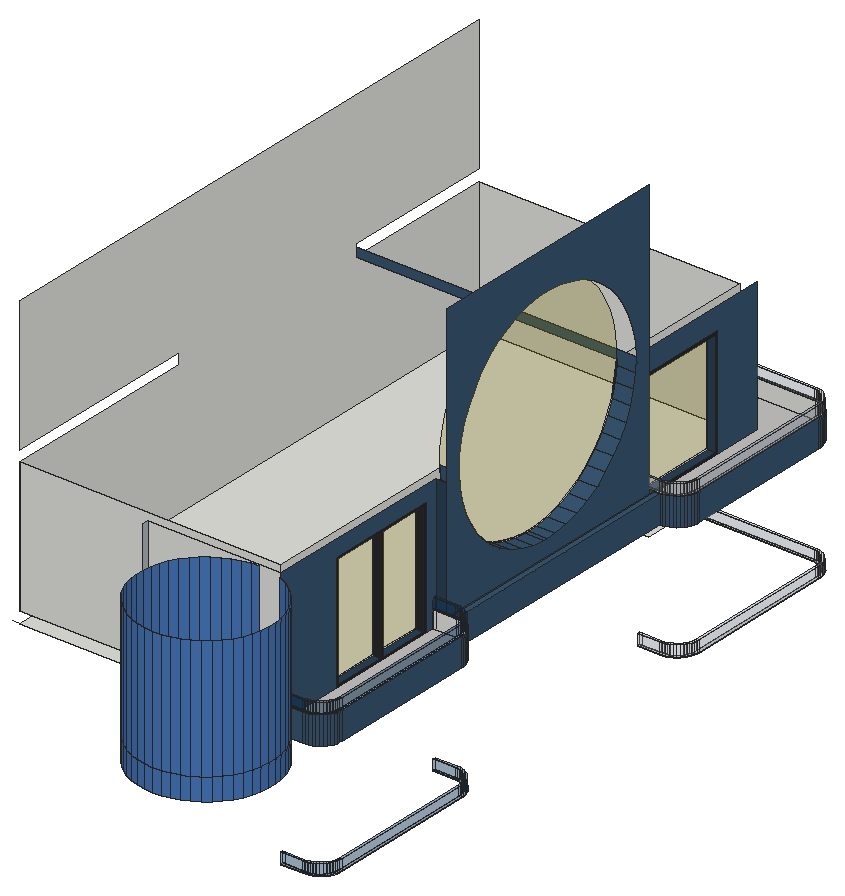
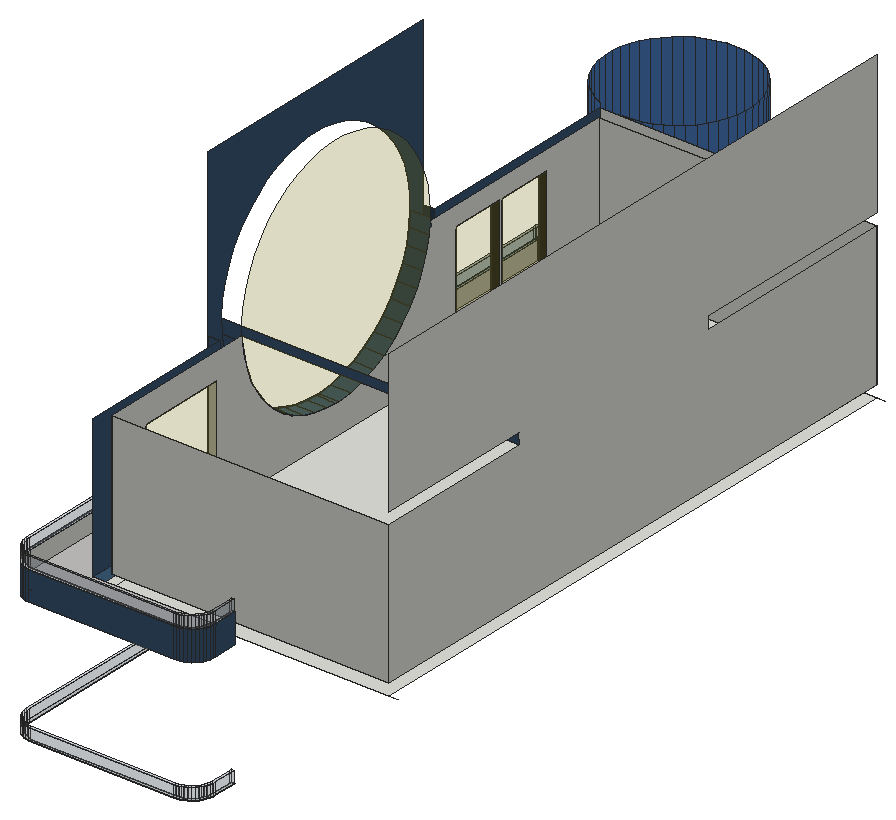
# SketchUp Ruby script. Lengths in inches.
U = 1.inch
M = Sketchup.active_model
def pt(a) = Geom::Point3d.new(a.map { |v| v * U })
def face(e, loops, mat)
  f = e.add_face(loops[0].map { |a| pt(a) })
  loops[1..].each { |l| e.add_face(l.map { |a| pt(a) }).erase! }
  f.material = f.back_material = mat if mat
  f
end
# faces: each face lists its corners as indices into pts; further lists are holes
def faces(e, pts, list, mat = nil) = list.each { |f| face(e, (f[0].is_a?(Array) ? f : [f]).map { |l| l.map { |i| pts[i] } }, mat) }
# xy, xz, yz: faces in a plane at the given z, y or x. An outline is a flat list of corners, or four numbers for a rectangle; further outlines are holes
def ring(l) = l.size == 4 ? [[l[0], l[1]], [l[2], l[1]], [l[2], l[3]], [l[0], l[3]]] : l.each_slice(2).to_a
def flat(e, list, mat, &to3) = list.each { |f| face(e, (f[0].is_a?(Array) ? f : [f]).map { |l| ring(l).map { |u, v| to3.(u, v) } }, mat) }
def xy(e, z, list, mat = nil) = flat(e, list, mat) { |x, y| [x, y, z] }
def xz(e, y, list, mat = nil) = flat(e, list, mat) { |x, z| [x, y, z] }
def yz(e, x, list, mat = nil) = flat(e, list, mat) { |y, z| [x, y, z] }
def lines(e, pts, list) = list.each { |a, b| e.add_line(pt(pts[a]), pt(pts[b])) }
# prism: a flat outline (further loops are holes) pulled along v
def prism(e, loops, v, mat = nil)
  f = face(e, loops, mat); d = Geom::Vector3d.new(v.map { |x| x * U })
  f.pushpull(f.normal.samedirection?(d) ? d.length : -d.length)
end
def box(e, o, s, mat = nil) = prism(e, [[o, [o[0] + s[0], o[1], o[2]], [o[0] + s[0], o[1] + s[1], o[2]], [o[0], o[1] + s[1], o[2]]]], [0, 0, s[2]], mat)
def at(x, y, z, deg = 0) = Geom::Transformation.translation(pt([x, y, z])) * Geom::Transformation.rotation(ORIGIN, Z_AXIS, deg.degrees)
def axes(o, x, y, z) = Geom::Transformation.new([*x, 0, *y, 0, *z, 0, *pt(o).to_a, 1])
def part(name) = M.definitions.add(name)
# library, detail: a bought-in or finely detailed component or shape, given as its bounding box
def library(name, o, s) = part(name).tap { |d| box(d.entities, o, s) }
def detail(e, o, s) = box(e.add_group.entities, o, s)
def put(e, d, t, mat = nil) = e.add_instance(d, t).tap { |i| i.material = mat if mat }
def group(e, t, mat = nil) = e.add_group.tap { |g| g.transformation = t; g.material = mat if mat }.entities
root = M.entities
M.materials.add("Carpet_01_1K").color = [196, 195, 193]
M.materials.add("Carpet_04_1K").color = [56, 85, 112]
M.materials.add("Carpet_04_1K1").color = [43, 65, 85]
M.materials.add("Glass_Basic_01").color = [186, 175, 28]
M.materials["Glass_Basic_01"].alpha = 0.25
M.materials.add("Glass_Basic_1").color = [0, 47, 91]
M.materials["Glass_Basic_1"].alpha = 0.25
M.materials.add("Glass_Basic_2").color = [161, 173, 186]
M.materials["Glass_Basic_2"].alpha = 0.25
M.materials.add("Glass_Mirror_01").color = [71, 118, 185]
M.materials.add("ThomThom - Buttons2").color = [40, 40, 43]
c1 = part("Group\#1")
prism(c1.entities,[[[0,206.04,0],[0,209.04,0],[24,209.04,0],[24.001,209.04,0],[27.133,208.835,0],[30.212,208.222,0],[33.184,207.213,0],[36,205.825,0],[38.61,204.081,0],[40.971,202.011,0],[43.04,199.65,0],[44.785,197.04,0],[46.173,194.224,0],[47.182,191.252,0],[47.795,188.173,0],[48,185.04,0],[48,24,0],[47.795,20.867,0],[47.182,17.788,0],[46.602,16.08,0],[46.173,14.816,0],[44.785,12,0],[43.04,9.39,0],[40.971,7.029,0],[38.61,4.96,0],[36,3.215,0],[33.184,1.827,0],[30.212,0.818,0],[27.133,0.205,0],[24,0,0],[0,0,0],[0,3,0],[3,3,0],[24,3,0],[26.741,3.18,0],[29.435,3.716,0],[32.036,4.599,0],[34.5,5.814,0],[36.784,7.34,0],[38.849,9.151,0],[40.66,11.216,0],[42.187,13.5,0],[43.401,15.964,0],[44.284,18.565,0],[44.82,21.259,0],[45,24,0],[45,185.04,0],[44.82,187.781,0],[44.284,190.475,0],[43.401,193.076,0],[42.187,195.54,0],[40.66,197.824,0],[38.849,199.889,0],[36.784,201.701,0],[34.5,203.227,0],[32.036,204.442,0],[29.435,205.325,0],[26.741,205.86,0],[24,206.04,0],[3,206.04,0]]],[0,0,12])
c2 = part("Group\#2")
prism(c2.entities,[[[147,3,0],[168,3,0],[170.74,3.18,0],[173.44,3.72,0],[176.04,4.6,0],[178.5,5.8125,0],[180.78,7.34,0],[182.85,9.15,0],[184.66,11.22,0],[186.1875,13.5,0],[187.4,15.96,0],[188.28,18.56,0],[188.82,21.26,0],[189,24,0],[189,184.94,0],[188.8125,187.78,0],[188.28,190.47,0],[187.4,193.07,0],[186.18,195.54,0],[184.66,197.82,0],[182.84,199.88,0],[180.78,201.7,0],[178.5,203.22,0],[176.03,204.4375,0],[173.43,205.32,0],[171.01,205.8,0],[24,205.8,0],[21.26,205.62,0],[18.56,205.08,0],[15.96,204.2,0],[13.5,202.99,0],[11.22,201.46,0],[9.15,199.65,0],[7.34,197.58,0],[5.8125,195.3,0],[4.6,192.84,0],[3.72,190.24,0],[3.18,187.54,0],[3,184.8,0],[3,163.8,0],[3,160.8,0],[0,160.8,0],[0,184.8,0],[0.21,187.93,0],[0.82,191.01,0],[1.83,193.98,0],[3.22,196.8,0],[4.96,199.41,0],[7.03,201.77,0],[9.39,203.84,0],[12,205.58,0],[14.82,206.97,0],[17.79,207.98,0],[20.87,208.59,0],[24,208.8,0],[171.31,208.8,0],[174.21,208.22,0],[177.18,207.21,0],[180,205.82,0],[182.61,204.08,0],[184.97,202.01,0],[187.04,199.65,0],[188.78,197.04,0],[190.17,194.22,0],[191.18,191.25,0],[191.79,188.17,0],[192,185.04,0],[192,24,0],[191.79,20.87,0],[191.18,17.79,0],[190.17,14.82,0],[188.78,12,0],[187.04,9.39,0],[184.97,7.03,0],[182.61,4.96,0],[180,3.22,0],[177.18,1.83,0],[174.21,0.82,0],[171.13,0.21,0],[168,0,0],[144,0,0],[144,3,0]]],[0,0,12])
xy(root,948,[[330.57,155.5,354.57,155.5,357.71,155.71,360.79,156.32,363.76,157.33,366.57,158.72,369.19,160.46,371.55,162.53,373.62,164.89,375.36,167.5,376.75,170.32,377.76,173.29,378.37,176.37,378.57,179.5,378.57,340.54,378.37,343.67,377.76,346.75,376.75,349.73,375.36,352.54,373.62,355.15,371.55,357.51,369.19,359.58,366.57,361.33,363.76,362.71,360.79,363.72,357.71,364.34,354.57,364.54,330.57,364.54,330.57,361.54,354.57,361.54,357.32,361.36,360.01,360.83,362.61,359.94,365.07,358.73,367.36,357.2,369.42,355.39,371.24,353.33,372.76,351.04,373.98,348.58,374.86,345.98,375.4,343.28,375.57,340.54,375.57,179.5,375.4,176.76,374.86,174.07,373.98,171.46,372.76,169,371.24,166.72,369.42,164.65,367.36,162.84,365.07,161.31,362.61,160.1,360.01,159.22,357.32,158.68,354.57,158.5,330.57,158.5],[330.57,637.9,354.57,637.9,357.71,638.11,360.79,638.72,363.76,639.73,366.57,641.12,369.19,642.86,371.55,644.93,373.62,647.29,375.36,649.9,376.75,652.72,377.76,655.6875,378.37,658.77,378.57,661.9,378.57,822.94,378.37,826.07,377.76,829.15,376.75,832.125,375.36,834.94,373.62,837.55,371.55,839.91,369.19,841.98,366.57,843.73,363.76,845.11,360.79,846.12,357.88,846.7,210.57,846.7,207.44,846.5,204.36,845.88,201.39,844.875,198.57,843.49,195.96,841.74,193.6,839.67,191.53,837.3125,189.79,834.7,188.4,831.89,187.39,828.91,186.78,825.83,186.57,822.7,186.57,798.7,189.57,798.7,189.57,822.7,189.75,825.44,190.29,828.14,191.17,830.74,192.39,833.2,193.91,835.48,195.73,837.55,197.79,839.36,200.07,840.89,202.54,842.1,205.14,842.99,207.83,843.52,210.57,843.7,357.59,843.7,360.01,843.22,362.61,842.34,365.07,841.12,367.36,839.6,369.42,837.79,371.23,835.72,372.76,833.4375,373.97,830.97,374.85,828.375,375.39,825.68,375.57,822.84,375.57,661.9,375.4,659.16,374.86,656.47,373.98,653.86,372.76,651.4,371.24,649.12,369.42,647.05,367.36,645.24,365.07,643.71,362.61,642.5,360.01,641.62,357.32,641.08,354.57,640.9,330.57,640.9]])
xy(root,1047,[[321.57,652.9,330.57,742.9]])
xy(root,1054,[[321.57,233.15,330.57,291.15],[321.57,293.15,330.57,349.15]],"ThomThom - Buttons2")
xy(root,1067,[[321.57,419.54,330.57,500.22],[321.57,502.22,330.57,582.9]])
xy(root,1074,[[39.57,167.5625,321.57,786.64],[321.57,167.5625,330.57,786.64]])
xy(root,1074,[[330.57,155.5,330.57,364.54,354.57,364.54,357.71,364.34,360.79,363.72,363.76,362.71,366.57,361.33,369.19,359.58,371.55,357.51,373.62,355.15,375.36,352.54,376.75,349.73,377.76,346.75,378.37,343.67,378.57,340.54,378.57,179.5,378.37,176.37,377.76,173.29,376.75,170.32,375.36,167.5,373.62,164.89,371.55,162.53,369.19,160.46,366.57,158.72,363.76,157.33,360.79,156.32,357.71,155.71,354.57,155.5],[330.57,364.54,354.57,637.9],[330.57,637.9,330.57,798.7,186.57,798.7,186.57,822.7,186.78,825.83,187.39,828.91,188.4,831.89,189.79,834.7,191.53,837.3125,193.6,839.67,195.96,841.74,198.57,843.49,201.39,844.875,204.36,845.88,207.44,846.5,210.57,846.7,357.88,846.7,360.79,846.12,363.76,845.11,366.57,843.73,369.19,841.98,371.55,839.91,373.62,837.55,375.36,834.94,376.75,832.125,377.76,829.15,378.37,826.07,378.57,822.94,378.57,661.9,378.37,658.77,377.76,655.6875,376.75,652.72,375.36,649.9,373.62,647.29,371.55,644.93,369.19,642.86,366.57,641.12,363.76,639.73,360.79,638.72,357.71,638.11,354.57,637.9]],"Carpet_04_1K")
xy(root,1086,[[39.57,167.5625,321.57,786.64]])
xy(root,1086,[[330.57,158.5,354.57,158.5,357.32,158.68,360.01,159.22,362.61,160.1,365.07,161.31,367.36,162.84,369.42,164.65,371.24,166.72,372.76,169,373.98,171.46,374.86,174.07,375.4,176.76,375.57,179.5,375.57,340.54,375.4,343.28,374.86,345.98,373.98,348.58,372.76,351.04,371.24,353.33,369.42,355.39,367.36,357.2,365.07,358.73,362.61,359.94,360.01,360.83,357.32,361.36,354.57,361.54,330.57,361.54],[330.57,640.9,354.57,640.9,357.32,641.08,360.01,641.62,362.61,642.5,365.07,643.71,367.36,645.24,369.42,647.05,371.24,649.12,372.76,651.4,373.98,653.86,374.86,656.47,375.4,659.16,375.57,661.9,375.57,822.84,375.39,825.68,374.85,828.375,373.97,830.97,372.76,833.4375,371.23,835.72,369.42,837.79,367.36,839.6,365.07,841.12,362.61,842.34,360.01,843.22,357.59,843.7,210.57,843.7,207.83,843.52,205.14,842.99,202.54,842.1,200.07,840.89,197.79,839.36,195.73,837.55,193.91,835.48,192.39,833.2,191.17,830.74,190.29,828.14,189.75,825.44,189.57,822.7,189.57,798.7,330.57,798.7]],"Carpet_01_1K")
xy(root,1086,[[342.57,364.54,348.57,637.9]],"Carpet_04_1K")
xy(root,1088,[[321.57,233.15,330.57,291.15],[321.57,293.15,330.57,349.15]],"Carpet_04_1K1")
xy(root,1089,[[321.57,652.9,330.57,742.9]],"Carpet_04_1K1")
xy(root,1104,[[330.57,155.5,354.57,155.5,357.71,155.71,360.79,156.32,363.76,157.33,366.57,158.72,369.19,160.46,371.55,162.53,373.62,164.89,375.36,167.5,376.75,170.32,377.76,173.29,378.37,176.37,378.57,179.5,378.57,340.54,378.37,343.67,377.76,346.75,376.75,349.73,375.36,352.54,373.62,355.15,371.55,357.51,369.19,359.58,366.57,361.33,363.76,362.71,360.79,363.72,357.71,364.34,354.57,364.54,330.57,364.54,330.57,361.54,354.57,361.54,357.32,361.36,360.01,360.83,362.61,359.94,365.07,358.73,367.36,357.2,369.42,355.39,371.24,353.33,372.76,351.04,373.98,348.58,374.86,345.98,375.4,343.28,375.57,340.54,375.57,179.5,375.4,176.76,374.86,174.07,373.98,171.46,372.76,169,371.24,166.72,369.42,164.65,367.36,162.84,365.07,161.31,362.61,160.1,360.01,159.22,357.32,158.68,354.57,158.5,330.57,158.5],[330.57,637.9,354.57,637.9,357.71,638.11,360.79,638.72,363.76,639.73,366.57,641.12,369.19,642.86,371.55,644.93,373.62,647.29,375.36,649.9,376.75,652.72,377.76,655.6875,378.37,658.77,378.57,661.9,378.57,822.94,378.37,826.07,377.76,829.15,376.75,832.125,375.36,834.94,373.62,837.55,371.55,839.91,369.19,841.98,366.57,843.73,363.76,845.11,360.79,846.12,357.88,846.7,210.57,846.7,207.44,846.5,204.36,845.88,201.39,844.875,198.57,843.49,195.96,841.74,193.6,839.67,191.53,837.3125,189.79,834.7,188.4,831.89,187.39,828.91,186.78,825.83,186.57,822.7,186.57,798.7,189.57,798.7,189.57,822.7,189.75,825.44,190.29,828.14,191.17,830.74,192.39,833.2,193.91,835.48,195.73,837.55,197.79,839.36,200.07,840.89,202.54,842.1,205.14,842.99,207.83,843.52,210.57,843.7,357.59,843.7,360.01,843.22,362.61,842.34,365.07,841.12,367.36,839.6,369.42,837.79,371.23,835.72,372.76,833.4375,373.97,830.97,374.85,828.375,375.39,825.68,375.57,822.84,375.57,661.9,375.4,659.16,374.86,656.47,373.98,653.86,372.76,651.4,371.24,649.12,369.42,647.05,367.36,645.24,365.07,643.71,362.61,642.5,360.01,641.62,357.32,641.08,354.57,640.9,330.57,640.9]])
xy(root,1104,[[348.57,364.54,354.57,637.9]],"Carpet_04_1K")
xy(root,1203,[[321.57,652.9,330.57,742.9]])
xy(root,1210,[[321.57,233.15,330.57,291.15],[321.57,293.15,330.57,349.15]])
xz(root,155.5,[[186.57,1074,330.57,1086],[186.57,1086,330.57,1230]])
xz(root,155.5,[[330.57,1074,354.57,1104]],"Carpet_04_1K")
xz(root,158.5,[[330.57,1086,333.57,1104],[333.57,1086,354.57,1104]])
xz(root,167.5625,[[39.57,1086,321.57,1230]])
xz(root,233.15,[[321.57,1088,330.57,1210]],"ThomThom - Buttons2")
xz(root,291.15,[[321.57,1088,330.57,1210]],"ThomThom - Buttons2")
xz(root,293.15,[[321.57,1088,330.57,1210]],"ThomThom - Buttons2")
xz(root,349.15,[[321.57,1088,330.57,1210]],"ThomThom - Buttons2")
xz(root,361.54,[[330.57,1086,333.57,1104],[333.57,1086,354.57,1104]])
xz(root,364.54,[[330.57,1086,342.57,1104]])
xz(root,364.54,[[342.57,1086,348.57,1104]],"Carpet_04_1K")
xz(root,364.54,[[330.57,1104,342.57,1230]],"Carpet_04_1K1")
xz(root,637.9,[[330.57,1086,342.57,1104]])
xz(root,637.9,[[342.57,1086,348.57,1104],[330.57,1104,342.57,1230]],"Carpet_04_1K")
xz(root,640.9,[[330.57,1086,333.57,1104],[333.57,1086,354.57,1104]])
xz(root,652.9,[[321.57,1089,330.57,1203]])
xz(root,742.9,[[321.57,1089,330.57,1203]],"Carpet_04_1K1")
xz(root,786.64,[[39.57,1086,321.57,1230]])
xz(root,798.7,[[186.57,1086,189.57,1104]])
xz(root,843.7,[[210.57,1086,357.59,1104]])
xz(root,846.7,[[210.57,1074,357.88,1104]],"Carpet_04_1K")
yz(root,39.57,[[167.5625,1086,786.64,1086,786.64,1230,620.85,1230,621.17,1239.34,620.93,1242,786.64,1242,786.64,1386,167.5625,1386,167.5625,1242,381.59,1242,381.51,1230,167.5625,1230]])
yz(root,186.57,[[149.51,1074,155.5,1086],[149.51,1086,155.5,1230]],"Carpet_01_1K")
yz(root,186.57,[[798.7,1074,822.7,1104]],"Carpet_04_1K")
yz(root,189.57,[[798.7,1086,801.7,1104],[801.7,1086,822.7,1104]])
yz(root,236.92,[[77.22,1074,86.26,1098],[77.22,1098,86.26,1230]],"Glass_Mirror_01")
yz(root,321.57,[[[167.5625,1086,167.5625,1230,381.51,1230,382.63,1217.66,385.87,1202.9375,390.92,1188.74,397.71,1175.29,406.14,1162.79,416.0625,1151.45,427.33,1141.45,439.76,1132.93,453.17,1126.04,467.33,1120.89,482.02,1117.55,497.02,1116.07,501.22,1116.19,512.08,1116.49,526.98,1118.8,541.46,1122.95,555.3125,1128.88,568.3125,1136.51,580.25,1145.7,590.95,1156.32,600.23,1168.19,607.94,1181.14,613.98,1194.94,618.24,1209.4,620.65,1224.28,620.85,1230,786.64,1230,786.64,1086],[652.9,1089,742.9,1203],[233.15,1088,291.15,1210],[293.15,1088,349.15,1210]]])
yz(root,321.57,[[233.15,1088,291.15,1210],[293.15,1088,349.15,1210],[652.9,1089,742.9,1203],[497.02,1116.07,482.02,1117.55,467.33,1120.89,453.17,1126.04,439.76,1132.93,427.33,1141.45,416.0625,1151.45,406.14,1162.79,397.71,1175.29,390.92,1188.74,385.87,1202.9375,382.63,1217.66,381.51,1230,381.59,1242,381.8,1247.72,384.21,1262.6,388.46,1277.06,394.5,1290.86,402.22,1303.81,411.49,1315.68,422.1875,1326.3,434.13,1335.49,447.13,1343.12,460.98,1349.05,475.47,1353.2,490.36,1355.51,501.22,1355.81,505.42,1355.93,520.42,1354.45,535.12,1351.11,549.28,1345.96,562.68,1339.07,575.11,1330.55,586.38,1320.55,596.3,1309.21,604.73,1296.71,611.52,1283.26,616.58,1269.0625,619.8125,1254.34,620.93,1242,620.93,1232.43,613.98,1194.94,607.94,1181.14,600.23,1168.19,590.95,1156.32,580.25,1145.7,568.3125,1136.51,555.3125,1128.88,541.46,1122.95,526.98,1118.8,512.08,1116.49,501.22,1116.19]],"Glass_Basic_01")
yz(root,330.57,[[155.5,1086,158.5,1104],[361.54,1086,364.54,1104],[637.9,1086,640.9,1104]])
yz(root,330.57,[[158.5,1086,231.15,1086,231.15,1212,351.15,1212,351.15,1086,361.54,1086,361.54,1104,364.54,1104,364.54,1230,155.5,1230,155.5,1104,158.5,1104],[640.9,1086,649.9,1086,649.9,1206,745.9,1206,745.9,1086,798.7,1086,798.7,1230,637.9,1230,637.9,1104,640.9,1104]],"Carpet_04_1K")
yz(root,330.57,[[[231.15,1086,351.15,1212],[233.15,1088,233.15,1210,349.15,1210,349.15,1088,293.15,1088,293.15,1210,291.15,1210,291.15,1088]],[[649.9,1086,745.9,1206],[652.9,1089,742.9,1203]]],"ThomThom - Buttons2")
yz(root,342.57,[[[364.54,1086,637.9,1398],[497.02,1116.07,482.02,1117.55,467.33,1120.89,453.17,1126.04,439.76,1132.93,427.33,1141.45,416.0625,1151.45,406.14,1162.79,397.71,1175.29,390.92,1188.74,385.87,1202.9375,382.63,1217.66,381.27,1232.66,381.8,1247.72,384.21,1262.6,388.46,1277.06,394.5,1290.86,402.22,1303.81,411.49,1315.68,422.1875,1326.3,434.13,1335.49,447.13,1343.12,460.98,1349.05,475.47,1353.2,490.36,1355.51,501.22,1355.81,505.42,1355.93,520.42,1354.45,535.12,1351.11,549.28,1345.96,562.68,1339.07,575.11,1330.55,586.38,1320.55,596.3,1309.21,604.73,1296.71,611.52,1283.26,616.58,1269.0625,619.8125,1254.34,621.17,1239.34,620.65,1224.28,618.24,1209.4,613.98,1194.94,607.94,1181.14,600.23,1168.19,590.95,1156.32,580.25,1145.7,568.3125,1136.51,555.3125,1128.88,541.46,1122.95,526.98,1118.8,512.08,1116.49,501.22,1116.19]]],"Carpet_04_1K")
yz(root,348.57,[[364.54,1086,637.9,1104]],"Carpet_04_1K")
yz(root,354.57,[[364.54,1074,637.9,1104]],"Carpet_04_1K")
yz(root,375.57,[[179.5,1086,340.54,1104],[661.9,1086,822.84,1104]])
yz(root,378.57,[[179.5,1074,340.54,1104],[661.9,1074,822.94,1104]],"Carpet_04_1K")
yz(root,380.64,[[77.22,1074,86.26,1098],[77.22,1098,86.26,1230]],"Glass_Mirror_01")
p = [[308.78,9.74,1074],[308.78,9.74,1098],[299.76,10.31,1098],[299.76,10.31,1074],[317.8,10.31,1074],[317.8,10.31,1098],
  [290.875,12,1098],[290.875,12,1074],[326.6875,12,1074],[326.6875,12,1098],[282.28,14.79,1098],[282.28,14.79,1074],
  [335.29,14.79,1074],[335.29,14.79,1098],[274.09,18.64,1098],[274.09,18.64,1074],[343.47,18.64,1074],[343.47,18.64,1098],
  [266.46,23.49,1098],[266.46,23.49,1074],[351.1,23.49,1074],[351.1,23.49,1098],[259.49,29.25,1098],[259.49,29.25,1074],
  [358.07,29.25,1074],[358.07,29.25,1098],[253.3,35.84,1098],[253.3,35.84,1074],[364.26,35.84,1074],[364.26,35.84,1098],
  [247.99,43.16,1098],[247.99,43.16,1074],[369.57,43.16,1074],[369.57,43.16,1098],[243.63,51.08,1098],[243.63,51.08,1074],
  [373.93,51.08,1074],[373.93,51.08,1098],[240.3,59.49,1098],[240.3,59.49,1074],[377.26,59.49,1074],[377.26,59.49,1098],
  [238.06,68.25,1098],[238.06,68.25,1074],[379.51,68.25,1074],[379.51,68.25,1098],[236.92,77.22,1098],[236.92,77.22,1074],
  [380.64,77.22,1074],[380.64,77.22,1098],[236.92,86.26,1074],[236.92,86.26,1098],[238.06,95.23,1098],[238.06,95.23,1074],
  [379.51,95.23,1074],[379.51,95.23,1098],[380.64,86.26,1098],[380.64,86.26,1074],[240.3,103.99,1098],[240.3,103.99,1074],
  [377.26,103.99,1074],[377.26,103.99,1098],[243.63,112.39,1098],[243.63,112.39,1074],[373.93,112.39,1074],[373.93,112.39,1098],
  [247.99,120.32,1098],[247.99,120.32,1074],[369.57,120.32,1074],[369.57,120.32,1098],[253.3,127.63,1098],[253.3,127.63,1074],
  [364.26,127.63,1074],[364.26,127.63,1098],[259.49,134.22,1098],[259.49,134.22,1074],[358.07,134.22,1074],[358.07,134.22,1098],
  [266.46,139.99,1098],[266.46,139.99,1074],[351.1,139.99,1074],[351.1,139.99,1098],[274.09,144.83,1098],[274.09,144.83,1074],
  [343.47,144.83,1074],[343.47,144.83,1098],[282.28,148.68,1098],[282.28,148.68,1074],[335.29,148.68,1074],[335.29,148.68,1098],
  [290.875,151.48,1098],[290.875,151.48,1074],[299.76,153.17,1098],[299.76,153.17,1074],[308.78,153.74,1098],[308.78,153.74,1074],
  [357.71,155.71,1074],[357.71,155.71,1104],[354.57,155.5,1104],[354.57,155.5,1074],[360.79,156.32,1074],[360.79,156.32,1104],
  [363.76,157.33,1074],[363.76,157.33,1104],[366.57,158.72,1074],[366.57,158.72,1104],[369.19,160.46,1074],[369.19,160.46,1104],
  [371.55,162.53,1074],[371.55,162.53,1104],[373.62,164.89,1074],[373.62,164.89,1104],[375.36,167.5,1074],[375.36,167.5,1104],
  [376.75,170.32,1074],[376.75,170.32,1104],[377.76,173.29,1074],[377.76,173.29,1104],[378.37,176.37,1074],[378.37,176.37,1104],
  [378.57,179.5,1074],[378.57,179.5,1104],[378.37,343.67,1074],[378.37,343.67,1104],[378.57,340.54,1104],[378.57,340.54,1074],
  [377.76,346.75,1074],[377.76,346.75,1104],[376.75,349.73,1074],[376.75,349.73,1104],[375.36,352.54,1074],[375.36,352.54,1104],
  [373.62,355.15,1074],[373.62,355.15,1104],[371.55,357.51,1074],[371.55,357.51,1104],[369.19,359.58,1074],[369.19,359.58,1104],
  [366.57,361.33,1074],[366.57,361.33,1104],[363.76,362.71,1074],[363.76,362.71,1104],[360.79,363.72,1074],[360.79,363.72,1104],
  [357.71,364.34,1074],[357.71,364.34,1104],[354.57,364.54,1074],[354.57,364.54,1104],[357.71,638.11,1074],[357.71,638.11,1104],
  [354.57,637.9,1104],[354.57,637.9,1074],[360.79,638.72,1074],[360.79,638.72,1104],[363.76,639.73,1074],[363.76,639.73,1104],
  [366.57,641.12,1074],[366.57,641.12,1104],[369.19,642.86,1074],[369.19,642.86,1104],[371.55,644.93,1074],[371.55,644.93,1104],
  [373.62,647.29,1074],[373.62,647.29,1104],[375.36,649.9,1074],[375.36,649.9,1104],[376.75,652.72,1074],[376.75,652.72,1104],
  [377.76,655.6875,1074],[377.76,655.6875,1104],[378.37,658.77,1074],[378.37,658.77,1104],[378.57,661.9,1074],[378.57,661.9,1104],
  [186.57,822.7,1074],[186.57,822.7,1104],[186.78,825.83,1104],[186.78,825.83,1074],[378.37,826.07,1074],[378.37,826.07,1104],
  [378.57,822.94,1104],[378.57,822.94,1074],[187.39,828.91,1104],[187.39,828.91,1074],[377.76,829.15,1074],[377.76,829.15,1104],
  [188.4,831.89,1104],[188.4,831.89,1074],[376.75,832.125,1074],[376.75,832.125,1104],[189.79,834.7,1104],[189.79,834.7,1074],
  [375.36,834.94,1074],[375.36,834.94,1104],[191.53,837.3125,1104],[191.53,837.3125,1074],[373.62,837.55,1074],[373.62,837.55,1104],
  [193.6,839.67,1104],[193.6,839.67,1074],[371.55,839.91,1074],[371.55,839.91,1104],[195.96,841.74,1104],[195.96,841.74,1074],
  [369.19,841.98,1074],[369.19,841.98,1104],[198.57,843.49,1104],[198.57,843.49,1074],[366.57,843.73,1074],[366.57,843.73,1104],
  [201.39,844.875,1104],[201.39,844.875,1074],[363.76,845.11,1074],[363.76,845.11,1104],[204.36,845.88,1104],[204.36,845.88,1074],
  [360.79,846.12,1074],[360.79,846.12,1104],[207.44,846.5,1104],[207.44,846.5,1074],[357.88,846.7,1086],[357.88,846.7,1104],
  [357.88,846.7,1074],[210.57,846.7,1104],[210.57,846.7,1074],[357.32,158.68,1086],[354.57,158.5,1086],[354.57,158.5,1104],
  [357.32,158.68,1104],[360.01,159.22,1086],[360.01,159.22,1104],[362.61,160.1,1086],[362.61,160.1,1104],[365.07,161.31,1086],
  [365.07,161.31,1104],[367.36,162.84,1086],[367.36,162.84,1104],[369.42,164.65,1086],[369.42,164.65,1104],[371.24,166.72,1086],
  [371.24,166.72,1104],[372.76,169,1086],[372.76,169,1104],[373.98,171.46,1086],[373.98,171.46,1104],[374.86,174.07,1086],
  [374.86,174.07,1104],[375.4,176.76,1086],[375.4,176.76,1104],[375.57,179.5,1086],[375.57,179.5,1104],[375.4,343.28,1086],
  [375.57,340.54,1086],[375.57,340.54,1104],[375.4,343.28,1104],[374.86,345.98,1086],[374.86,345.98,1104],[373.98,348.58,1086],
  [373.98,348.58,1104],[372.76,351.04,1086],[372.76,351.04,1104],[371.24,353.33,1086],[371.24,353.33,1104],[369.42,355.39,1086],
  [369.42,355.39,1104],[367.36,357.2,1086],[367.36,357.2,1104],[365.07,358.73,1086],[365.07,358.73,1104],[362.61,359.94,1086],
  [362.61,359.94,1104],[360.01,360.83,1086],[360.01,360.83,1104],[357.32,361.36,1086],[357.32,361.36,1104],[354.57,361.54,1086],
  [354.57,361.54,1104],[357.32,641.08,1086],[354.57,640.9,1086],[354.57,640.9,1104],[357.32,641.08,1104],[360.01,641.62,1086],
  [360.01,641.62,1104],[362.61,642.5,1086],[362.61,642.5,1104],[365.07,643.71,1086],[365.07,643.71,1104],[367.36,645.24,1086],
  [367.36,645.24,1104],[369.42,647.05,1086],[369.42,647.05,1104],[371.24,649.12,1086],[371.24,649.12,1104],[372.76,651.4,1086],
  [372.76,651.4,1104],[373.98,653.86,1086],[373.98,653.86,1104],[374.86,656.47,1086],[374.86,656.47,1104],[375.4,659.16,1086],
  [375.4,659.16,1104],[375.57,661.9,1086],[375.57,661.9,1104],[189.57,822.7,1086],[189.75,825.44,1086],[189.75,825.44,1104],
  [189.57,822.7,1104],[375.39,825.68,1086],[375.57,822.84,1086],[375.57,822.84,1104],[375.39,825.68,1104],[190.29,828.14,1086],
  [190.29,828.14,1104],[374.85,828.375,1086],[374.85,828.375,1104],[191.17,830.74,1086],[191.17,830.74,1104],[373.97,830.97,1086],
  [373.97,830.97,1104],[192.39,833.2,1086],[192.39,833.2,1104],[372.76,833.4375,1086],[372.76,833.4375,1104],[193.91,835.48,1086],
  [193.91,835.48,1104],[371.23,835.72,1086],[371.23,835.72,1104],[195.73,837.55,1086],[195.73,837.55,1104],[369.42,837.79,1086],
  [369.42,837.79,1104],[197.79,839.36,1086],[197.79,839.36,1104],[367.36,839.6,1086],[367.36,839.6,1104],[200.07,840.89,1086],
  [200.07,840.89,1104],[365.07,841.12,1086],[365.07,841.12,1104],[202.54,842.1,1086],[202.54,842.1,1104],[362.61,842.34,1086],
  [362.61,842.34,1104],[205.14,842.99,1086],[205.14,842.99,1104],[360.01,843.22,1086],[360.01,843.22,1104],[207.83,843.52,1086],
  [207.83,843.52,1104],[357.59,843.7,1086],[357.59,843.7,1104],[210.57,843.7,1086],[210.57,843.7,1104],[299.76,10.31,1230],
  [308.78,9.74,1230],[317.8,10.31,1230],[290.875,12,1230],[326.6875,12,1230],[282.28,14.79,1230],[335.29,14.79,1230],
  [274.09,18.64,1230],[343.47,18.64,1230],[266.46,23.49,1230],[351.1,23.49,1230],[259.49,29.25,1230],[358.07,29.25,1230],
  [253.3,35.84,1230],[364.26,35.84,1230],[247.99,43.16,1230],[369.57,43.16,1230],[243.63,51.08,1230],[373.93,51.08,1230],
  [240.3,59.49,1230],[377.26,59.49,1230],[238.06,68.25,1230],[379.51,68.25,1230],[236.92,77.22,1230],[380.64,77.22,1230],
  [238.06,95.23,1230],[236.92,86.26,1230],[380.64,86.26,1230],[379.51,95.23,1230],[240.3,103.99,1230],[377.26,103.99,1230],
  [243.63,112.39,1230],[373.93,112.39,1230],[247.99,120.32,1230],[369.57,120.32,1230],[253.3,127.63,1230],[364.26,127.63,1230],
  [259.49,134.22,1230],[358.07,134.22,1230],[266.46,139.99,1230],[351.1,139.99,1230],[274.09,144.83,1230],[343.47,144.83,1230],
  [282.28,148.68,1230],[335.29,148.68,1230],[290.875,151.48,1230],[299.76,153.17,1230],[308.78,153.74,1230],[321.57,482.02,1117.55],
  [342.57,482.02,1117.55],[342.57,497.02,1116.07],[321.57,497.02,1116.07],[342.57,501.22,1116.19],[321.57,501.22,1116.19],[342.57,512.08,1116.49],
  [321.57,512.08,1116.49],[342.57,526.98,1118.8],[321.57,526.98,1118.8],[321.57,467.33,1120.89],[342.57,467.33,1120.89],[342.57,541.46,1122.95],
  [321.57,541.46,1122.95],[321.57,453.17,1126.04],[342.57,453.17,1126.04],[342.57,555.3125,1128.88],[321.57,555.3125,1128.88],[321.57,439.76,1132.93],
  [342.57,439.76,1132.93],[342.57,568.3125,1136.51],[321.57,568.3125,1136.51],[321.57,427.33,1141.45],[342.57,427.33,1141.45],[342.57,580.25,1145.7],
  [321.57,580.25,1145.7],[321.57,416.0625,1151.45],[342.57,416.0625,1151.45],[342.57,590.95,1156.32],[321.57,590.95,1156.32],[321.57,406.14,1162.79],
  [342.57,406.14,1162.79],[342.57,600.23,1168.19],[321.57,600.23,1168.19],[321.57,397.71,1175.29],[342.57,397.71,1175.29],[342.57,607.94,1181.14],
  [321.57,607.94,1181.14],[321.57,390.92,1188.74],[342.57,390.92,1188.74],[342.57,613.98,1194.94],[321.57,613.98,1194.94],[321.57,385.87,1202.9375],
  [342.57,385.87,1202.9375],[342.57,618.24,1209.4],[321.57,618.24,1209.4],[321.57,382.63,1217.66],[342.57,382.63,1217.66],[342.57,620.65,1224.28],
  [321.57,620.65,1224.28],[321.57,381.27,1232.66],[342.57,381.27,1232.66],[321.57,381.51,1230],[342.57,621.17,1239.34],[39.57,621.17,1239.34],
  [39.57,620.85,1230],[321.57,620.85,1230],[39.57,786.64,1074],[30.57,786.64,1074],[39.57,167.5625,1074],[30.57,167.5625,1074],
  [357.71,846.74,1086],[354.57,846.94,1086],[330.57,150.21,1074],[330.57,150.21,1098]]
faces(root,p,[[0,1,2,3],[4,5,1,0],[3,2,6,7],[8,9,5,4],[7,6,10,11],[12,13,9,8],[11,10,14,15],[16,17,13,12],
  [15,14,18,19],[20,21,17,16],[19,18,22,23],[24,25,21,20],[23,22,26,27],[28,29,25,24],[27,26,30,31],[32,33,29,28],
  [31,30,34,35],[36,37,33,32],[35,34,38,39],[40,41,37,36],[39,38,42,43],[44,45,41,40],[43,42,46,47],[48,49,45,44],
  [50,51,52,53],[54,55,56,57],[53,52,58,59],[60,61,55,54],[59,58,62,63],[64,65,61,60],[63,62,66,67],[68,69,65,64],
  [67,66,70,71],[72,73,69,68],[71,70,74,75],[76,77,73,72],[75,74,78,79],[80,81,77,76],[79,78,82,83],[84,85,81,80],
  [83,82,86,87],[88,89,85,84],[87,86,90,91],[91,90,92,93],[93,92,94,95],[353,2,1,354],[354,1,5,355],[356,6,2,353],
  [355,5,9,357],[358,10,6,356],[357,9,13,359],[360,14,10,358],[359,13,17,361],[362,18,14,360],[361,17,21,363],[364,22,18,362],
  [363,21,25,365],[366,26,22,364],[365,25,29,367],[368,30,26,366],[367,29,33,369],[370,34,30,368],[369,33,37,371],[372,38,34,370],
  [371,37,41,373],[374,42,38,372],[373,41,45,375],[376,46,42,374],[375,45,49,377],[378,52,51,379],[380,56,55,381],[382,58,52,378],
  [381,55,61,383],[384,62,58,382],[383,61,65,385],[386,66,62,384],[385,65,69,387],[388,70,66,386],[387,69,73,389],[390,74,70,388],
  [389,73,77,391],[392,78,74,390],[391,77,81,393],[394,82,78,392],[393,81,85,395],[396,86,82,394],[395,85,89,397],[398,90,86,396],
  [399,92,90,398],[400,94,92,399]],"Glass_Mirror_01")
faces(root,p,[[96,97,98,99],[100,101,97,96],[102,103,101,100],[104,105,103,102],[106,107,105,104],[108,109,107,106],[110,111,109,108],[112,113,111,110],
  [114,115,113,112],[116,117,115,114],[118,119,117,116],[120,121,119,118],[122,123,124,125],[126,127,123,122],[128,129,127,126],[130,131,129,128],
  [132,133,131,130],[134,135,133,132],[136,137,135,134],[138,139,137,136],[140,141,139,138],[142,143,141,140],[144,145,143,142],[146,147,145,144],
  [148,149,150,151],[152,153,149,148],[154,155,153,152],[156,157,155,154],[158,159,157,156],[160,161,159,158],[162,163,161,160],[164,165,163,162],
  [166,167,165,164],[168,169,167,166],[170,171,169,168],[172,173,171,170],[174,175,176,177],[178,179,180,181],[177,176,182,183],[184,185,179,178],
  [183,182,186,187],[188,189,185,184],[187,186,190,191],[192,193,189,188],[191,190,194,195],[196,197,193,192],[195,194,198,199],[200,201,197,196],
  [199,198,202,203],[204,205,201,200],[203,202,206,207],[208,209,205,204],[207,206,210,211],[212,213,209,208],[211,210,214,215],[216,217,213,212],
  [215,214,218,219],[220,221,217,216,222],[219,218,223,224],[401,402,403,404],[404,403,405,406],[406,405,407,408],[408,407,409,410],[411,412,402,401],
  [410,409,413,414],[415,416,412,411],[414,413,417,418],[419,420,416,415],[418,417,421,422],[423,424,420,419],[422,421,425,426],[427,428,424,423],
  [426,425,429,430],[431,432,428,427],[430,429,433,434],[435,436,432,431],[434,433,437,438],[439,440,436,435],[438,437,441,442],[443,444,440,439],
  [442,441,445,446],[447,448,444,443],[446,445,449,450],[451,452,448,447,453],[450,449,454,455,456,457]],"Carpet_04_1K")
faces(root,p,[[225,226,227,228],[229,225,228,230],[231,229,230,232],[233,231,232,234],[235,233,234,236],[237,235,236,238],[239,237,238,240],[241,239,240,242],
  [243,241,242,244],[245,243,244,246],[247,245,246,248],[249,247,248,250],[251,252,253,254],[255,251,254,256],[257,255,256,258],[259,257,258,260],
  [261,259,260,262],[263,261,262,264],[265,263,264,266],[267,265,266,268],[269,267,268,270],[271,269,270,272],[273,271,272,274],[275,273,274,276],
  [277,278,279,280],[281,277,280,282],[283,281,282,284],[285,283,284,286],[287,285,286,288],[289,287,288,290],[291,289,290,292],[293,291,292,294],
  [295,293,294,296],[297,295,296,298],[299,297,298,300],[301,299,300,302],[303,304,305,306],[307,308,309,310],[304,311,312,305],[313,307,310,314],
  [311,315,316,312],[317,313,314,318],[315,319,320,316],[321,317,318,322],[319,323,324,320],[325,321,322,326],[323,327,328,324],[329,325,326,330],
  [327,331,332,328],[333,329,330,334],[331,335,336,332],[337,333,334,338],[335,339,340,336],[341,337,338,342],[339,343,344,340],[345,341,342,346],
  [343,347,348,344],[349,345,346,350],[347,351,352,348]])
lines(root,p,[[458,459],[460,461],[462,463],[220,462],[88,464],[89,465]])
put(root,c1,at(330.57,155.5,948),"Glass_Basic_1")
put(root,c2,at(186.57,637.9,948),"Glass_Basic_2")
put(root,c1,at(330.57,155.5,1104),"Glass_Basic_1")
put(root,c2,at(186.57,637.9,1104),"Glass_Basic_2")
